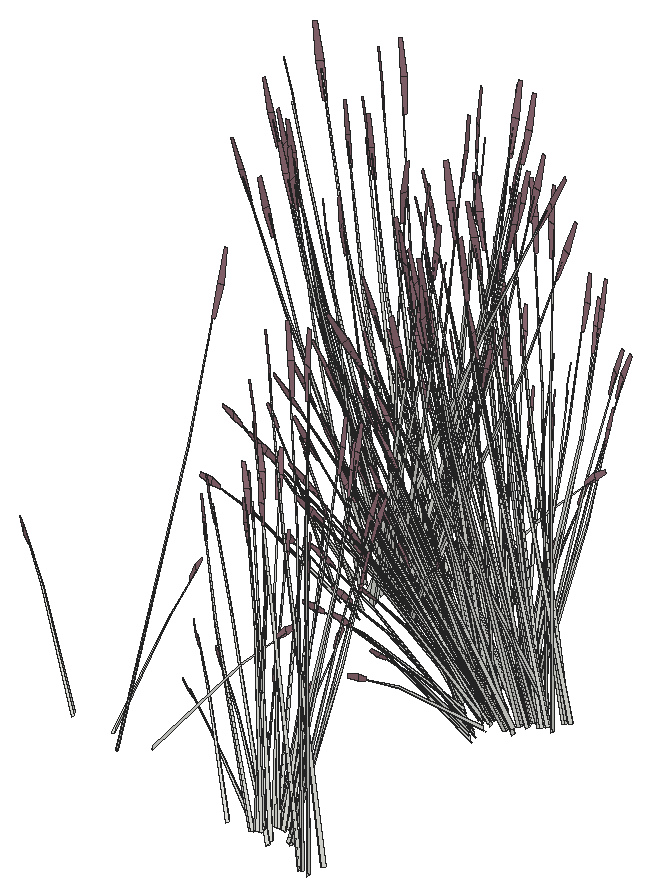
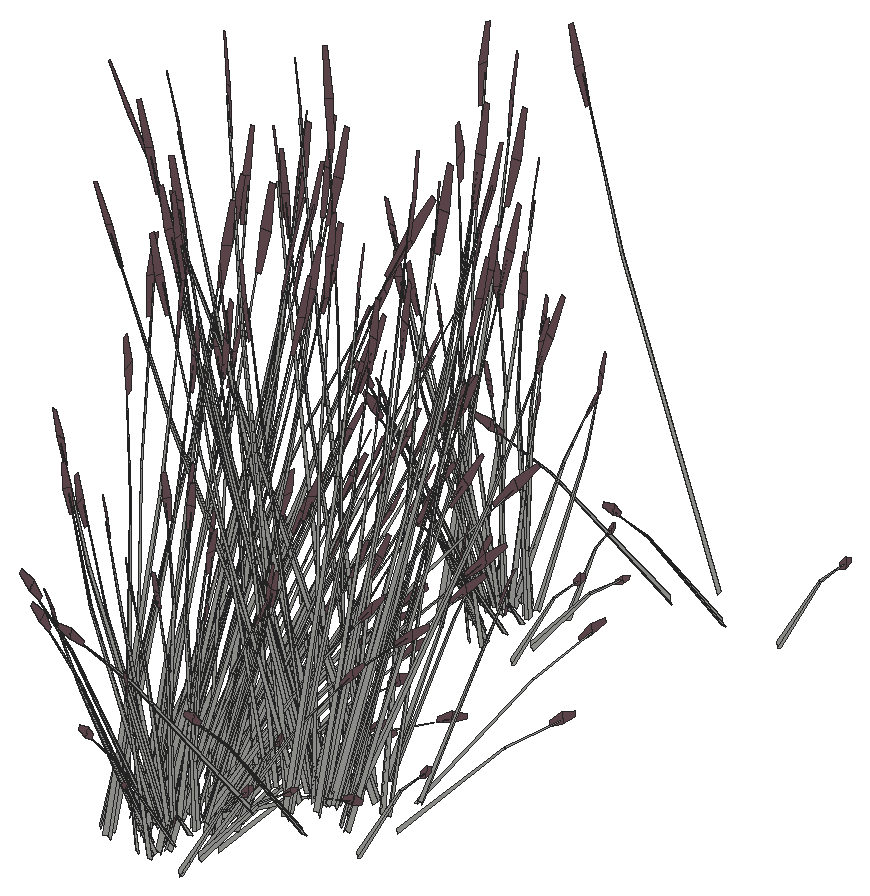
# SketchUp Ruby script. Lengths in inches.
U = 1.inch
M = Sketchup.active_model
def pt(a) = Geom::Point3d.new(a.map { |v| v * U })
def face(e, loops, mat)
  f = e.add_face(loops[0].map { |a| pt(a) })
  loops[1..].each { |l| e.add_face(l.map { |a| pt(a) }).erase! }
  f.material = f.back_material = mat if mat
  f
end
# faces: each face lists its corners as indices into pts; further lists are holes
def faces(e, pts, list, mat = nil) = list.each { |f| face(e, (f[0].is_a?(Array) ? f : [f]).map { |l| l.map { |i| pts[i] } }, mat) }
# xy, xz, yz: faces in a plane at the given z, y or x. An outline is a flat list of corners, or four numbers for a rectangle; further outlines are holes
def ring(l) = l.size == 4 ? [[l[0], l[1]], [l[2], l[1]], [l[2], l[3]], [l[0], l[3]]] : l.each_slice(2).to_a
def flat(e, list, mat, &to3) = list.each { |f| face(e, (f[0].is_a?(Array) ? f : [f]).map { |l| ring(l).map { |u, v| to3.(u, v) } }, mat) }
def xy(e, z, list, mat = nil) = flat(e, list, mat) { |x, y| [x, y, z] }
def xz(e, y, list, mat = nil) = flat(e, list, mat) { |x, z| [x, y, z] }
def yz(e, x, list, mat = nil) = flat(e, list, mat) { |y, z| [x, y, z] }
def lines(e, pts, list) = list.each { |a, b| e.add_line(pt(pts[a]), pt(pts[b])) }
# prism: a flat outline (further loops are holes) pulled along v
def prism(e, loops, v, mat = nil)
  f = face(e, loops, mat); d = Geom::Vector3d.new(v.map { |x| x * U })
  f.pushpull(f.normal.samedirection?(d) ? d.length : -d.length)
end
def box(e, o, s, mat = nil) = prism(e, [[o, [o[0] + s[0], o[1], o[2]], [o[0] + s[0], o[1] + s[1], o[2]], [o[0], o[1] + s[1], o[2]]]], [0, 0, s[2]], mat)
def at(x, y, z, deg = 0) = Geom::Transformation.translation(pt([x, y, z])) * Geom::Transformation.rotation(ORIGIN, Z_AXIS, deg.degrees)
def axes(o, x, y, z) = Geom::Transformation.new([*x, 0, *y, 0, *z, 0, *pt(o).to_a, 1])
def part(name) = M.definitions.add(name)
# library, detail: a bought-in or finely detailed component or shape, given as its bounding box
def library(name, o, s) = part(name).tap { |d| box(d.entities, o, s) }
def detail(e, o, s) = box(e.add_group.entities, o, s)
def put(e, d, t, mat = nil) = e.add_instance(d, t).tap { |i| i.material = mat if mat }
def group(e, t, mat = nil) = e.add_group.tap { |g| g.transformation = t; g.material = mat if mat }.entities
root = M.entities
M.materials.add("LightPink_Translucent").color = [144, 107, 117]
c1 = part("blade")
p = [[2.15,0.21,22],[0,0.17,0],[0.09,0.45,0],[2.18,0.31,22],[2.29,0.31,22],[0.38,0.45,0],
  [2.48,0.24,33],[2.49,0.24,33],[2.48,0.22,33]]
faces(c1.entities,p,[[0,1,2,3],[4,5,2,3],[6,3,4,7],[8,0,3,6]])
c2 = part("seeds")
p = [[0.3,-0.1,1.38],[-0.01,-0.03,1.59],[-0.01,-0.03,0.03],[0.14,-0.07,-0.07],[0.29,-0.03,3],[0.15,0.01,3.11]]
faces(c2.entities,p,[[0,1,2,3],[1,0,4,5]],"LightPink_Translucent")
c3 = part("blade with seeds")
put(c3.entities,c1,at(0,0,0))
put(c3.entities,c2,axes([2.4,0.25,30.99],[1.5799,-0.05474,1.17369],[-0.12525,1.92788,0.29478],[-0.07173,-0.02425,1.56792]))
put(root,c3,axes([46.08,647.97,43.49],[0.16438,0.10347,1.76342],[0.27873,0.95868,-0.26939],[-0.36432,0.20444,0.30037]))
put(root,c3,axes([50.95,687.73,43.49],[0.03108,0.16322,1.76342],[-0.62654,0.85237,-0.26939],[-0.44504,-0.04296,0.30037]))
put(root,c3,axes([50.62,692.3,43.49],[0.16438,0.10347,1.76342],[0.27873,0.95868,-0.26939],[-0.36432,0.20444,0.30037]))
put(root,c3,axes([55.05,689.21,44.06],[-1.27479,-0.1698,-0.62353],[0.26901,-1.04736,-0.16365],[-0.38043,-0.12691,1.37633]))
put(root,c3,axes([53.38,691.19,44.02],[-1.14694,-0.51783,-0.49651],[0.68554,-0.92854,0],[-0.26122,-0.11794,1.57504]))
put(root,c3,axes([52.875,683.48,43.49],[-0.11871,0.13643,1.76342],[-1.19964,0.29415,-0.26939],[-0.2898,-0.26759,0.30037]))
put(root,c3,axes([52.13,684,44.13],[-0.35352,0.84566,-0.03893],[-1.08806,-0.26014,-0.17649],[-0.1652,-0.13832,0.58215]))
put(root,c3,axes([56.5,689.36,44.67],[-1.23732,0.68758,-0.29095],[-0.8228,-0.97154,-0.50002],[-0.30528,-0.09867,1.59708]))
put(root,c3,axes([53.7,690.8,44.03],[-0.28787,-0.90242,-0.30978],[1.14332,-0.25625,0.30978],[-0.23049,-0.10406,1.38974]))
put(root,c3,axes([57.32,690.11,44.06],[-0.82544,0.77843,-0.62353],[-1.0254,-0.70586,-0.16365],[-0.33076,0.19418,1.37633]))
put(root,c3,axes([57.89,689.68,44.46],[-1.19666,-0.83357,-0.25192],[1.00694,-0.93603,0.5513],[-0.32224,0.09751,1.68216]))
put(root,c3,axes([55.71,688.875,44.21],[-0.73619,-0.86927,-0.44739],[1.11511,-0.61213,0.21531],[-0.23824,-0.10756,1.43643]))
put(root,c3,axes([57.28,689.5,44.21],[-1.33077,0.06393,-0.44739],[-0.12035,-1.06125,0.21531],[-0.23824,0.10756,1.43643]))
put(root,c3,axes([55.82,689.37,44.4375],[0.32481,-1.2272,-0.23429],[1.54007,0.21392,0.51271],[-0.26911,-0.16947,1.5644]))
put(root,c3,axes([58.68,692.24,44.02],[-1.14694,0.51783,-0.49651],[-0.68554,-0.92854,0],[-0.26122,0.11794,1.57504]))
put(root,c3,axes([51.89,687.08,44.02],[0,-1.03566,-0.49651],[1.37109,0,0],[0,-0.23588,1.57504]))
put(root,c3,axes([51.15,648.0625,43.49],[0.19833,-0.05635,1.76342],[1.19302,0.31018,-0.26939],[0.03489,0.3496,0.30037]))
put(root,c3,axes([58.41,691.83,44.03],[-1.14332,-0.25625,-0.30978],[0.28787,-0.90242,0.30978],[-0.23049,0.10406,1.38974]))
put(root,c3,axes([55.47,688.28,44.67],[-1.38012,-0.49416,-0.29095],[0.66454,-1.04299,-0.50002],[-0.04337,-0.25608,1.59708]))
put(root,c3,axes([58.22,689.21,44.67],[0.1428,1.18174,-0.29095],[-1.48733,0.07145,-0.50002],[-0.26191,0.15741,1.59708]))
put(root,c3,axes([54.86,687.23,44.1],[-0.50328,-1.06202,-0.69835],[1.44974,-0.38248,-0.18329],[-0.05563,-0.35963,1.54149]))
put(root,c3,axes([52.48,687.1,44.03],[0.85545,-0.64616,-0.30978],[0.85545,0.64616,0.30978],[0,-0.20813,1.38974]))
put(root,c3,axes([56.34,682.92,44.13],[-0.84686,0.59414,-0.03893],[-0.77596,-0.65071,-0.17649],[-0.05463,-0.18438,0.58215]))
put(root,c3,axes([54.92,644.7,44.09],[0.44936,0.94823,-0.69212],[-1.29441,0.3415,-0.18165],[0.04967,0.32109,1.52773]))
put(root,c3,axes([56.55,682.19,43.49],[-0.20555,0.03731,1.76342],[-1.13672,-0.42002,-0.26939],[0.01907,-0.35034,0.30037]))
put(root,c3,axes([55.62,687.5,44.21],[0.59459,-0.93321,-0.44739],[1.23546,0.44912,0.21531],[0,-0.21512,1.43643]))
put(root,c3,axes([55.69,692.39,43.49],[0.19833,-0.05635,1.76342],[1.19302,0.31018,-0.26939],[0.03489,0.3496,0.30037]))
put(root,c3,axes([69.75,684.64,36.97],[0.50831,-0.02346,1.71376],[-0.33721,1.01661,0.13857],[-0.72439,-0.06288,0.73262]))
put(root,c3,axes([58.76,688.75,44.21],[-0.59459,0.93321,-0.44739],[-1.23546,-0.44912,0.21531],[0,0.21512,1.43643]))
put(root,c3,axes([69.96,686.43,36.97],[0.42521,-0.21906,1.71376],[0.35798,1.01226,0.13857],[-0.66754,0.22878,0.73262]))
put(root,c3,axes([68.64,688.16,35.68],[0.42589,0.08502,1.43002],[0.2745,0.86839,-0.30754],[-0.57851,0.16255,0.61141]))
put(root,c3,axes([72.41,685.375,36.43],[0.34834,-0.14982,1.77064],[0.12012,1.04605,0.13857],[-0.75452,0.1388,0.63284]))
put(root,c3,axes([68.66,686.08,37.81],[-0.20012,0.13446,1.74944],[0.01702,0.98243,-0.27667],[-0.45871,0.12776,0.14031]))
put(root,c3,axes([71.27,683.7,38.07],[-1.22504,-0.02494,-0.71045],[0.08228,-1.05005,0.08574],[-0.51899,-0.11081,1.00501]))
put(root,c3,axes([70.29,683.95,35.68],[0.23927,0.28834,1.43002],[-0.55135,0.78376,-0.30754],[-0.56612,-0.18733,0.61141]))
put(root,c3,axes([69.31,685.52,37.62],[-1.01846,-0.28891,-0.35414],[0.29705,-0.84289,0.4572],[-0.41005,0.07729,0.87481]))
put(root,c3,axes([61.9,689.15,44.03],[-0.85545,0.64616,-0.30978],[-0.85545,-0.64616,0.30978],[0,0.20813,1.38974]))
put(root,c3,axes([70.71,683.01,36.97],[0.45521,0.17844,1.71376],[-0.94204,0.74856,0.13857],[-0.58713,-0.33769,0.73262]))
put(root,c3,axes([59.46,689.03,44.09],[0.44936,0.94823,-0.69212],[-1.29441,0.3415,-0.18165],[0.04967,0.32109,1.52773]))
put(root,c3,axes([66.4375,647.51,38.5],[0.1564,0.02778,1.77383],[0.48382,0.91506,-0.16761],[-0.32016,0.24017,0.31391]))
put(root,c3,axes([66.4375,687.07,37.8],[0.1564,0.02778,1.77383],[0.48382,0.91506,-0.16761],[-0.32016,0.24017,0.31391]))
put(root,c3,axes([70,685.95,37.77],[-0.332,0.94205,-0.51099],[-1.13828,-0.3229,-0.3958],[-0.45829,0.08638,0.97773]))
put(root,c3,axes([56.16,687.04,44.67],[-0.1428,-1.18174,-0.29095],[1.48733,-0.07145,-0.50002],[0.26191,-0.15741,1.59708]))
put(root,c3,axes([70.87,683.91,37.77],[-0.88986,0.68603,-0.51099],[-0.77932,-0.72471,-0.3958],[-0.45212,-0.10438,0.97773]))
put(root,c3,axes([69.43,685.89,34.58],[0.03108,0.16322,1.76342],[-0.62654,0.85237,-0.26939],[-0.44504,-0.04296,0.30037]))
put(root,c3,axes([58.91,687.97,44.67],[1.38012,0.49416,-0.29095],[-0.66454,1.04299,-0.50002],[0.04337,0.25608,1.59708]))
put(root,c3,axes([69.61,681.99,37.8],[0.09085,0.10335,1.77383],[-0.43798,0.92907,-0.16761],[-0.44357,0.00672,0.31391]))
put(root,c3,axes([55.97,684.42,44.03],[1.14332,0.25625,-0.30978],[-0.28787,0.90242,0.30978],[0.23049,-0.10406,1.38974]))
put(root,c3,axes([67.75,650.42,36.56],[0.51072,-0.46938,1.1486],[0.20153,0.74307,0.84392],[-0.36908,0.13305,0.25299]))
put(root,c3,axes([67.75,689.98,35.86],[0.51072,-0.46938,1.1486],[0.20153,0.74307,0.84392],[-0.36908,0.13305,0.25299]))
put(root,c3,axes([70.625,681.37,37.81],[-0.26368,-0.00731,1.74944],[-0.83946,0.73103,-0.27667],[-0.44791,-0.14937,0.14031]))
put(root,c3,axes([69.54,685.41,37.82],[0.34623,-0.9443,0.48003],[1.13828,0.3229,0.3958],[-0.44763,0.05675,0.9933]))
put(root,c3,axes([62.49,689.17,44.02],[0,1.03566,-0.49651],[-1.37109,0,0],[0,0.23588,1.57504]))
put(root,c3,axes([55.7,684.01,44.02],[1.14694,-0.51783,-0.49651],[0.68554,0.92854,0],[0.26122,-0.11794,1.57504]))
put(root,c3,axes([69.95,685.14,38.125],[0.6166,0.93779,-0.1216],[-1.09436,0.46085,-0.67495],[-0.46117,0.12373,1.02557]))
put(root,c3,axes([71.33,683.19,38.125],[-0.06562,1.05324,-0.1216],[-1.2424,-0.02879,-0.67495],[-0.4785,-0.07316,1.02557]))
put(root,c3,axes([70.54,683.26,37.62],[-0.69728,-0.64842,-0.35414],[0.79619,-0.61382,0.4572],[-0.40453,-0.09339,0.87481]))
put(root,c3,axes([69.46,685.16,37.82],[-0.4501,-0.70615,0.0643],[0.82077,-0.34564,0.50621],[-0.36181,0.0682,0.77189]))
put(root,c3,axes([71.52,647.56,37.67],[0.30609,-0.31822,1.71376],[0.77286,0.85893,0.13857],[-0.53009,0.39116,0.73262]))
put(root,c3,axes([71.52,687.11,36.97],[0.30609,-0.31822,1.71376],[0.77286,0.85893,0.13857],[-0.53009,0.39116,0.73262]))
put(root,c3,axes([69.68,648.39,38.32],[-1.06674,0.14801,-0.35414],[-0.28168,-0.84611,0.4572],[-0.30569,0.22726,0.87481]))
put(root,c3,axes([69.68,687.95,37.62],[-1.06674,0.14801,-0.35414],[-0.28168,-0.84611,0.4572],[-0.30569,0.22726,0.87481]))
put(root,c3,axes([69.1,650.9,35.29],[0.16438,0.10347,1.76342],[0.27873,0.95868,-0.26939],[-0.36432,0.20444,0.30037]))
put(root,c3,axes([69.1,690.46,34.58],[0.16438,0.10347,1.76342],[0.27873,0.95868,-0.26939],[-0.36432,0.20444,0.30037]))
put(root,c3,axes([68.86,684.82,35.86],[0.78239,-0.07411,1.1486],[-0.49629,0.65296,0.84392],[-0.38663,-0.09795,0.25299]))
put(root,c3,axes([56.4,648.1,43.49],[0.08928,-0.14952,1.76342],[1.12407,-0.44035,-0.26939],[0.34078,0.22791,0.30037]))
put(root,c3,axes([58.64,690.38,44.18],[1.2866,-0.3514,-0.19198],[0.45209,1.01223,0.00008],[0.14202,-0.03884,1.73897]))
put(root,c3,axes([69.82,687.76,37.82],[-0.30393,-0.95317,0.48003],[1.19224,-0.16542,0.3958],[-0.35138,0.22417,0.9933]))
put(root,c3,axes([70.43,683.02,38.18],[1.01205,-0.7643,0.53763],[0.87284,0.81167,0.4433],[-0.47482,-0.14098,1.11249]))
put(root,c3,axes([69.58,687.58,37.82],[-0.8413,-0.43556,0.0643],[0.48981,-0.62025,0.50621],[-0.26973,0.20053,0.77189]))
put(root,c3,axes([58.67,687.375,44.21],[0.73619,0.86927,-0.44739],[-1.11511,0.61213,0.21531],[0.23824,0.10756,1.43643]))
put(root,c3,axes([71.29,648.34,37.67],[0.22818,-0.35597,1.71376],[0.95725,0.73667,0.13857],[-0.43183,0.45914,0.73262]))
put(root,c3,axes([71.29,687.9,36.97],[0.22818,-0.35597,1.71376],[0.95725,0.73667,0.13857],[-0.43183,0.45914,0.73262]))
put(root,c3,axes([70.38,685.42,38.14],[1.01846,0.28891,0.35414],[-0.29705,0.84289,-0.4572],[-0.41005,0.07729,0.87481]))
put(root,c3,axes([57.06,686.14,44.06],[0.82544,-0.77843,-0.62353],[1.0254,0.70586,-0.16365],[0.33076,-0.19418,1.37633]))
put(root,c3,axes([70.56,648.49,38.47],[0.31482,0.94565,-0.51099],[-1.19224,0.16542,-0.3958],[-0.34166,0.254,0.97773]))
put(root,c3,axes([70.56,688.04,37.77],[0.31482,0.94565,-0.51099],[-1.19224,0.16542,-0.3958],[-0.34166,0.254,0.97773]))
put(root,c3,axes([70.89,683.02,37.82],[0.06171,-0.78753,0.0643],[0.9318,0.02159,0.50621],[-0.35694,-0.08241,0.77189]))
put(root,c3,axes([68.7,650.1875,38.51],[-0.03046,0.20495,1.74944],[0.86449,0.71297,-0.27667],[-0.22632,0.33716,0.14031]))
put(root,c3,axes([68.7,689.74,37.81],[-0.03046,0.20495,1.74944],[0.86449,0.71297,-0.27667],[-0.22632,0.33716,0.14031]))
put(root,c3,axes([73.53,687.37,35.15],[-1.27479,-0.1698,-0.62353],[0.26901,-1.04736,-0.16365],[-0.38043,-0.12691,1.37633]))
put(root,c3,axes([73.76,681.65,38.52],[-0.81789,0.99285,-0.13619],[-1.18445,-0.572,-0.75594],[-0.41173,-0.28051,1.14864]))
put(root,c3,axes([60.68,685.44,44.03],[0.28787,0.90242,-0.30978],[-1.14332,0.25625,0.30978],[0.23049,0.10406,1.38974]))
put(root,c3,axes([71.53,683.6,38.14],[0.69728,0.64842,0.35414],[-0.79619,0.61382,-0.4572],[-0.40453,-0.09339,0.87481]))
put(root,c3,axes([73.4,682.46,38.07],[-1.04497,-0.50058,-0.71045],[0.74264,-0.8772,0.08574],[-0.3786,-0.29889,1.00501]))
put(root,c3,axes([72.91,682.48,37.77],[-1.20928,0.24619,-0.51099],[-0.21154,-0.93233,-0.3958],[-0.32481,-0.26718,0.97773]))
put(root,c3,axes([57.88,686.89,44.67],[1.23732,-0.68758,-0.29095],[0.8228,0.97154,-0.50002],[0.30528,0.09867,1.59708]))
put(root,c3,axes([71.86,689.35,35.11],[-1.14694,-0.51783,-0.49651],[0.68554,-0.92854,0],[-0.26122,-0.11794,1.57504]))
put(root,c3,axes([71.35,681.64,34.58],[-0.11871,0.13643,1.76342],[-1.19964,0.29415,-0.26939],[-0.2898,-0.26759,0.30037]))
put(root,c3,axes([70,647.8125,38.83],[1.1336,0.57106,-0.1216],[-0.65308,0.827,-0.67495],[-0.32027,0.28747,1.02557]))
put(root,c3,axes([70,687.37,38.125],[1.1336,0.57106,-0.1216],[-0.65308,0.827,-0.67495],[-0.32027,0.28747,1.02557]))
put(root,c3,axes([72.56,689.97,35.46],[-0.7662,1.03778,0],[-1.28187,-0.57875,-0.51607],[-0.29196,-0.13181,1.63711]))
put(root,c3,axes([54.76,686.27,43.59],[-1.20625,0.41464,1.28929],[-0.38394,-1.1897,0.50096],[0.74071,0.01979,1.46642]))
put(root,c3,axes([68.125,650.29,39.44],[1.08141,0.27645,-0.06488],[-0.33265,0.85086,-0.29416],[-0.17688,0.12919,0.97024]))
put(root,c3,axes([68.125,689.85,38.74],[1.08141,0.27645,-0.06488],[-0.33265,0.85086,-0.29416],[-0.17688,0.12919,0.97024]))
put(root,c3,axes([70.55,647.89,38.84],[1.06674,-0.14801,0.35414],[0.28168,0.84611,-0.4572],[-0.30569,0.22726,0.87481]))
put(root,c3,axes([70.55,687.45,38.14],[1.06674,-0.14801,0.35414],[0.28168,0.84611,-0.4572],[-0.30569,0.22726,0.87481]))
put(root,c3,axes([71.16,651.92,36.38],[0.38672,-0.16338,1.43002],[0.95481,0.49262,-0.30754],[-0.28419,0.42626,0.61141]))
put(root,c3,axes([71.16,691.48,35.68],[0.38672,-0.16338,1.43002],[0.95481,0.49262,-0.30754],[-0.28419,0.42626,0.61141]))
put(root,c3,axes([70.61,682.16,35.22],[-0.35352,0.84566,-0.03893],[-1.08806,-0.26014,-0.17649],[-0.1652,-0.13832,0.58215]))
put(root,c3,axes([61.58,683.98,43.49],[-0.18342,-0.08159,1.76342],[-0.47115,-0.9115,-0.26939],[0.31784,-0.24736,0.30037]))
put(root,c3,axes([73.44,679.29,37.8],[-0.02286,0.12414,1.77383],[-1.12758,0.45052,-0.16761],[-0.33182,-0.23029,0.31391]))
put(root,c3,axes([61,685.06,44.02],[1.14694,0.51783,-0.49651],[-0.68554,0.92854,0],[0.26122,0.11794,1.57504]))
put(root,c3,axes([72.23,681.1,35.68],[-0.07421,0.33879,1.43002],[-1.08488,0.28361,-0.30754],[-0.25359,-0.4379,0.61141]))
put(root,c3,axes([72.59,681.97,36.97],[0.28013,0.33252,1.71376],[-1.29445,0.27994,0.13857],[-0.29256,-0.52202,0.73262]))
put(root,c3,axes([60.94,692.43,43.49],[0.08928,-0.14952,1.76342],[1.12407,-0.44035,-0.26939],[0.34078,0.22791,0.30037]))
put(root,c3,axes([74.98,687.52,35.76],[-1.23732,0.68758,-0.29095],[-0.8228,-0.97154,-0.50002],[-0.30528,-0.09867,1.59708]))
put(root,c3,axes([71.56,650.14,38.53],[-0.87265,-0.70663,0.48003],[0.92674,-0.60943,0.3958],[-0.16097,0.33153,0.9933]))
put(root,c3,axes([71.56,689.69,37.82],[-0.87265,-0.70663,0.48003],[0.92674,-0.60943,0.3958],[-0.16097,0.33153,0.9933]))
put(root,c3,axes([73.04,681.8,37.62],[-0.18927,-0.83419,-0.35414],[1.08199,-0.22027,0.4572],[-0.29062,-0.23905,0.87481]))
put(root,c3,axes([70.02,686.02,35.46],[-1.53239,0,0],[0,-1.1575,-0.51607],[0,-0.26363,1.63711]))
put(root,c3,axes([72.18,688.96,35.12],[-0.28787,-0.90242,-0.30978],[1.14332,-0.25625,0.30978],[-0.23049,-0.10406,1.38974]))
put(root,c3,axes([71.24,650.07,38.52],[-1.00708,-0.04826,0.0643],[0.02761,-0.72867,0.50621],[-0.10538,0.27912,0.77189]))
put(root,c3,axes([71.24,689.625,37.82],[-1.00708,-0.04826,0.0643],[0.02761,-0.72867,0.50621],[-0.10538,0.27912,0.77189]))
put(root,c3,axes([59.33,687.04,44.06],[1.27479,0.1698,-0.62353],[-0.26901,1.04736,-0.16365],[0.38043,0.12691,1.37633]))
put(root,c3,axes([71.55,650.35,38.32],[-0.82919,0.54528,-0.35414],[-0.78493,-0.62262,0.4572],[-0.11943,0.31634,0.87481]))
put(root,c3,axes([71.55,689.9,37.62],[-0.82919,0.54528,-0.35414],[-0.78493,-0.62262,0.4572],[-0.11943,0.31634,0.87481]))
put(root,c3,axes([64.75,687.66,44.26],[-0.75977,-0.66224,-0.06488],[0.83212,-0.6068,-0.29416],[0.23578,-0.04272,0.97024]))
put(root,c3,axes([75.8,648.72,35.85],[-0.82544,0.77843,-0.62353],[-1.0254,-0.70586,-0.16365],[-0.33076,0.19418,1.37633]))
put(root,c3,axes([75.8,688.27,35.15],[-0.82544,0.77843,-0.62353],[-1.0254,-0.70586,-0.16365],[-0.33076,0.19418,1.37633]))
put(root,c3,axes([73.68,682.48,38.14],[0.18927,0.83419,0.35414],[-1.08199,0.22027,-0.4572],[-0.29062,-0.23905,0.87481]))
put(root,c3,axes([68.6,652.29,38.5],[0.13903,-0.06253,1.77383],[1.14912,0.41591,-0.16761],[-0.027,0.34629,0.31391]))
put(root,c3,axes([68.6,691.84,37.8],[0.13903,-0.06253,1.77383],[1.14912,0.41591,-0.16761],[-0.027,0.34629,0.31391]))
put(root,c3,axes([71.21,685.72,35.42],[-1.1399,0.87071,0.30756],[-1.1406,-0.86155,-0.36492],[-0.03981,-0.24727,1.64885]))
put(root,c3,axes([75.9,688.12,36.42],[1.05902,0.41762,1.51261],[-1.03748,0.89969,0.59816],[-0.46471,-0.53324,1.26806]))
put(root,c3,axes([71.86,680.55,35.86],[0.63926,0.36046,1.1486],[-0.93099,0.21668,0.84392],[-0.1992,-0.27702,0.25299]))
put(root,c3,axes([76.37,687.83,35.56],[-1.19666,-0.83357,-0.25192],[1.00694,-0.93603,0.5513],[-0.32224,0.09751,1.68216]))
put(root,c3,axes([74.19,687.03,35.3],[-0.73619,-0.86927,-0.44739],[1.11511,-0.61213,0.21531],[-0.23824,-0.10756,1.43643]))
put(root,c3,axes([72.11,649.77,39.13],[-0.03189,0.95798,-0.7886],[-1.34277,-0.06434,0.09517],[-0.14171,0.40585,1.11556]))
put(root,c3,axes([72.11,689.33,38.43],[-0.03189,0.95798,-0.7886],[-1.34277,-0.06434,0.09517],[-0.14171,0.40585,1.11556]))
put(root,c3,axes([72.08,652.47,36.56],[-0.03171,-0.6158,1.1486],[0.7925,0.43922,0.84392],[-0.15586,0.29352,0.25299]))
put(root,c3,axes([72.08,692.02,35.86],[-0.03171,-0.6158,1.1486],[0.7925,0.43922,0.84392],[-0.15586,0.29352,0.25299]))
put(root,c3,axes([73.2,681.5,38.18],[1.36515,-0.26619,0.53763],[0.23692,1.04421,0.4433],[-0.32106,-0.30775,1.11249]))
put(root,c3,axes([75.76,687.66,35.3],[-1.33077,0.06393,-0.44739],[-0.12035,-1.06125,0.21531],[-0.23824,0.10756,1.43643]))
put(root,c3,axes([73.51,681.72,37.82],[0.55698,-0.6579,0.0643],[0.79316,0.38303,0.50621],[-0.25643,-0.21093,0.77189]))
put(root,c3,axes([73.22,689.43,35.57],[1.14694,0.51783,0.49651],[-0.68554,0.92854,0],[-0.26122,-0.11794,1.57504]))
put(root,c3,axes([71.66,651.12,37.16],[0.02693,-0.53464,1.54345],[1.21102,0.2824,0.21329],[-0.10493,0.5698,0.72882]))
put(root,c3,axes([71.66,690.68,36.45],[0.02693,-0.53464,1.54345],[1.21102,0.2824,0.21329],[-0.10493,0.5698,0.72882]))
put(root,c3,axes([74.3,687.53,35.53],[0.32481,-1.2272,-0.23429],[1.54007,0.21392,0.51271],[-0.26911,-0.16947,1.5644]))
put(root,c3,axes([74.86,687.82,35.71],[-0.23642,0.92427,0.1448],[-1.15506,-0.16044,-0.41347],[-0.21021,-0.09491,1.26744]))
put(root,c3,axes([74.73,679.77,37.81],[-0.18744,-0.14521,1.74944],[-1.25089,0.09206,-0.27667],[-0.19964,-0.34731,0.14031]))
put(root,c3,axes([77.16,650.84,35.8125],[-1.14694,0.51783,-0.49651],[-0.68554,-0.92854,0],[-0.26122,0.11794,1.57504]))
put(root,c3,axes([77.16,690.4,35.11],[-1.14694,0.51783,-0.49651],[-0.68554,-0.92854,0],[-0.26122,0.11794,1.57504]))
put(root,c3,axes([70.37,685.24,35.11],[0,-1.03566,-0.49651],[1.37109,0,0],[0,-0.23588,1.57504]))
put(root,c3,axes([70.95,686.2,35.57],[0,1.03566,0.49651],[-1.37109,0,0],[0,-0.23588,1.57504]))
put(root,c3,axes([77.23,690.12,35.28],[-0.75665,-1.04141,-0.05142],[1.28187,-0.57875,0.51607],[-0.31588,0.09915,1.6363]))
put(root,c3,axes([72.38,650.09,38.8],[0.87728,0.69587,-0.5672],[-0.92674,0.60943,-0.43934],[-0.13348,0.35356,1.08528]))
put(root,c3,axes([72.38,689.65,38.1],[0.87728,0.69587,-0.5672],[-0.92674,0.60943,-0.43934],[-0.13348,0.35356,1.08528]))
put(root,c3,axes([76.89,689.99,35.12],[-1.14332,-0.25625,-0.30978],[0.28787,-0.90242,0.30978],[-0.23049,0.10406,1.38974]))
put(root,c3,axes([71.99,649.58,38.84],[0.82919,-0.54528,0.35414],[0.78493,0.62262,-0.4572],[-0.11943,0.31634,0.87481]))
put(root,c3,axes([71.99,689.13,38.14],[0.82919,-0.54528,0.35414],[0.78493,0.62262,-0.4572],[-0.11943,0.31634,0.87481]))
put(root,c3,axes([73.95,686.43,35.76],[-1.38012,-0.49416,-0.29095],[0.66454,-1.04299,-0.50002],[-0.04337,-0.25608,1.59708]))
put(root,c3,axes([77.55,646.57,36.64],[-0.03348,-0.97511,1.41272],[1.51511,0.25277,0.59816],[-0.35835,0.53357,1.3335]))
put(root,c3,axes([77.55,686.13,35.93],[-0.03348,-0.97511,1.41272],[1.51511,0.25277,0.59816],[-0.35835,0.53357,1.3335]))
put(root,c3,axes([71.46,649.73,39.19],[1.34686,0.05131,-0.13498],[-0.03681,0.97156,-0.74919],[-0.09356,0.37418,1.13838]))
put(root,c3,axes([71.46,689.28,38.49],[1.34686,0.05131,-0.13498],[-0.03681,0.97156,-0.74919],[-0.09356,0.37418,1.13838]))
put(root,c3,axes([71.43,651.14,36.62],[1.11329,-0.1834,0.06507],[0.25594,0.73887,-0.86304],[-0.07058,0.37403,0.7736]))
put(root,c3,axes([71.43,690.69,35.91],[1.11329,-0.1834,0.06507],[0.25594,0.73887,-0.86304],[-0.07058,0.37403,0.7736]))
put(root,c3,axes([76.69,647.82,36.46],[0.1428,1.18174,-0.29095],[-1.48733,0.07145,-0.50002],[-0.26191,0.15741,1.59708]))
put(root,c3,axes([76.69,687.37,35.76],[0.1428,1.18174,-0.29095],[-1.48733,0.07145,-0.50002],[-0.26191,0.15741,1.59708]))
put(root,c3,axes([73.33,685.38,35.1875],[-0.50328,-1.06202,-0.69835],[1.44974,-0.38248,-0.18329],[-0.05563,-0.35963,1.54149]))
put(root,c3,axes([76.63,682.01,38.125],[-1.19922,0.48218,-0.1216],[-0.58932,-0.85579,-0.67495],[-0.15822,-0.36063,1.02557]))
put(root,c3,axes([75.6,682.05,37.77],[-1.20468,-0.25962,-0.51099],[0.41292,-0.89013,-0.3958],[-0.11046,-0.35838,0.97773]))
put(root,c3,axes([73.38,649.09,37.67],[-0.02999,-0.3975,1.71376],[1.30002,0.26369,0.13857],[-0.08041,0.56647,0.73262]))
put(root,c3,axes([73.38,688.65,36.97],[-0.02999,-0.3975,1.71376],[1.30002,0.26369,0.13857],[-0.08041,0.56647,0.73262]))
